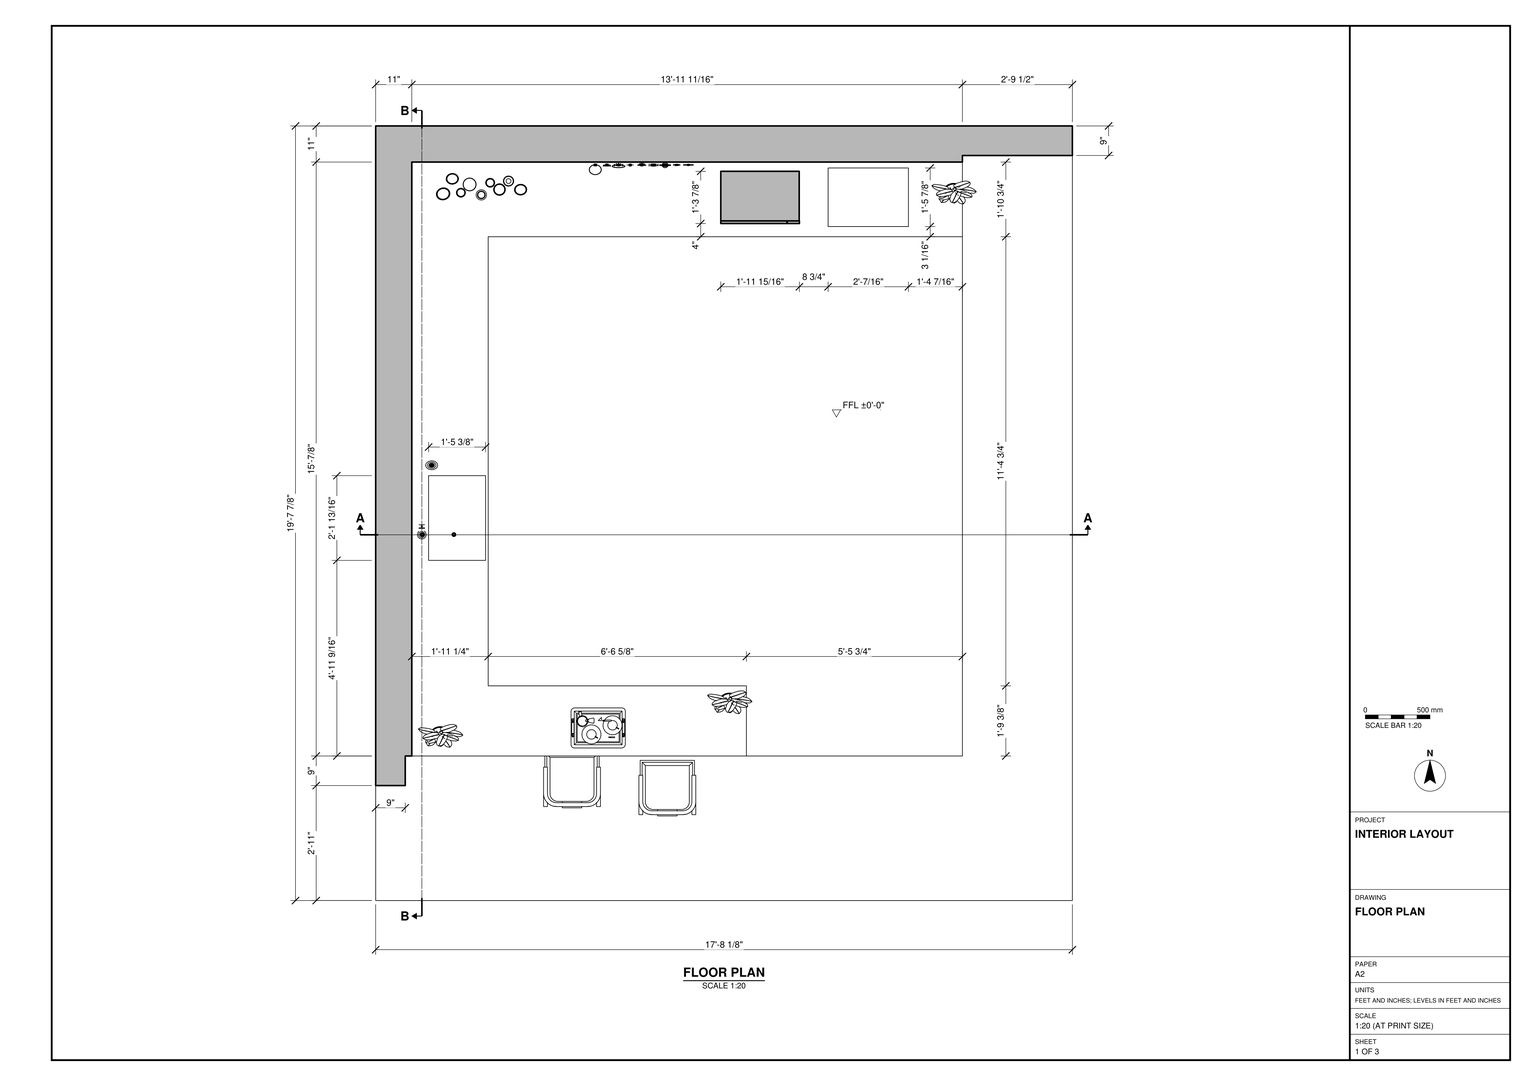
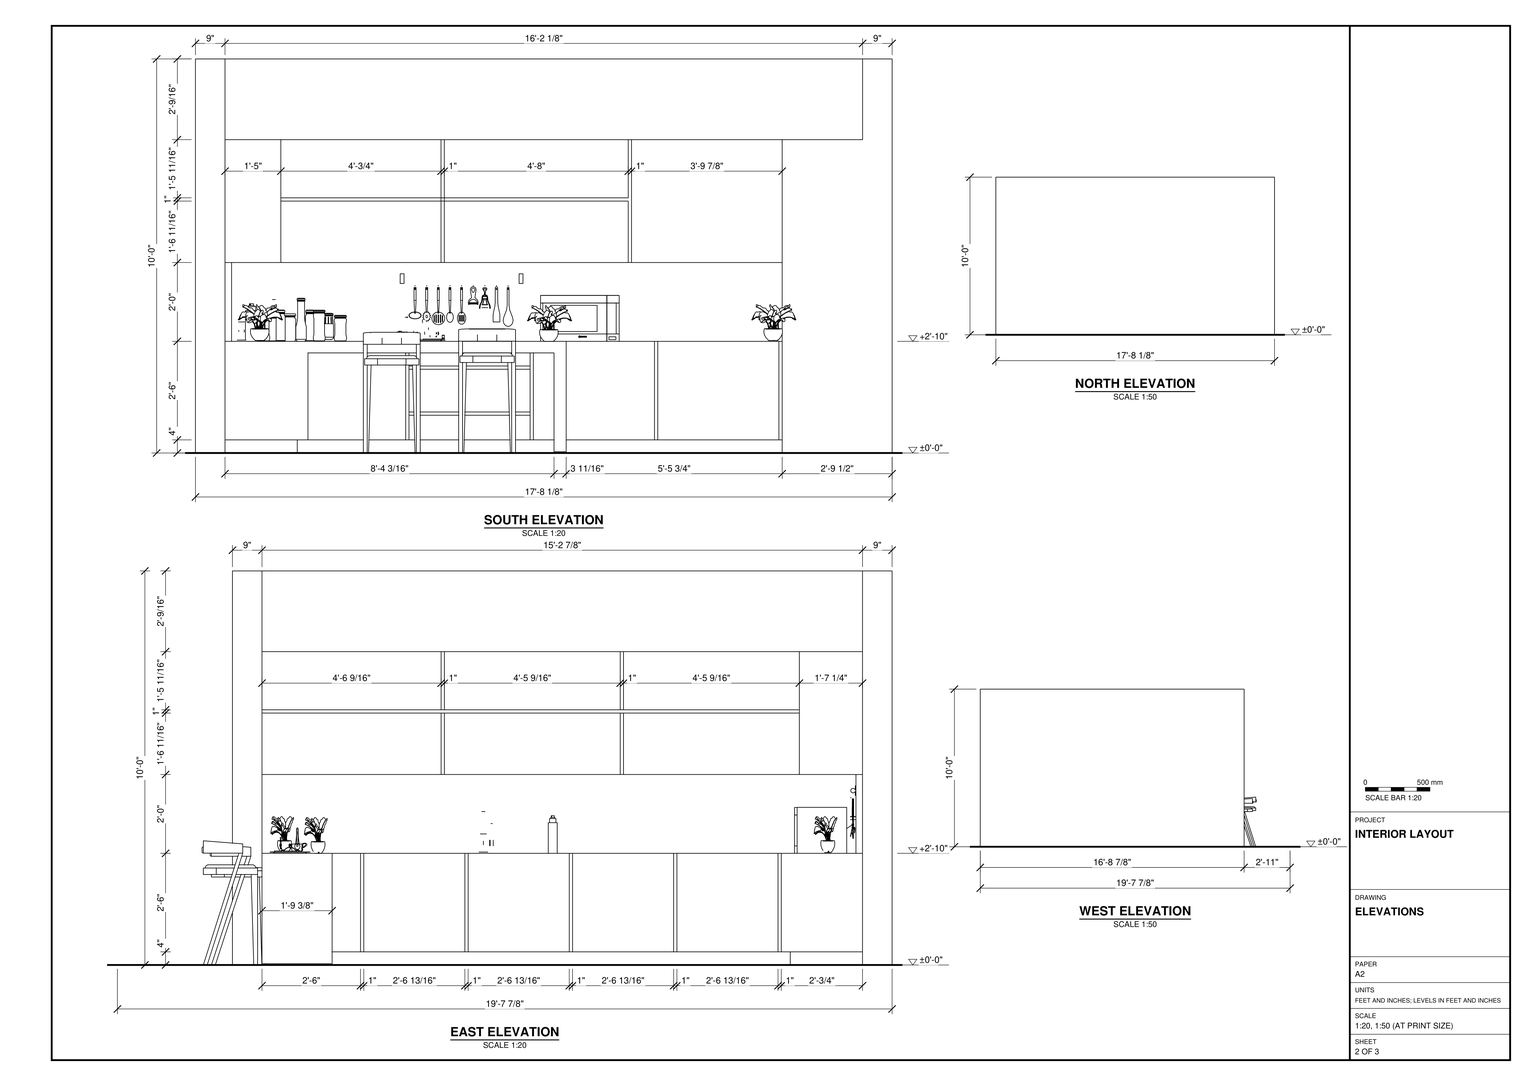
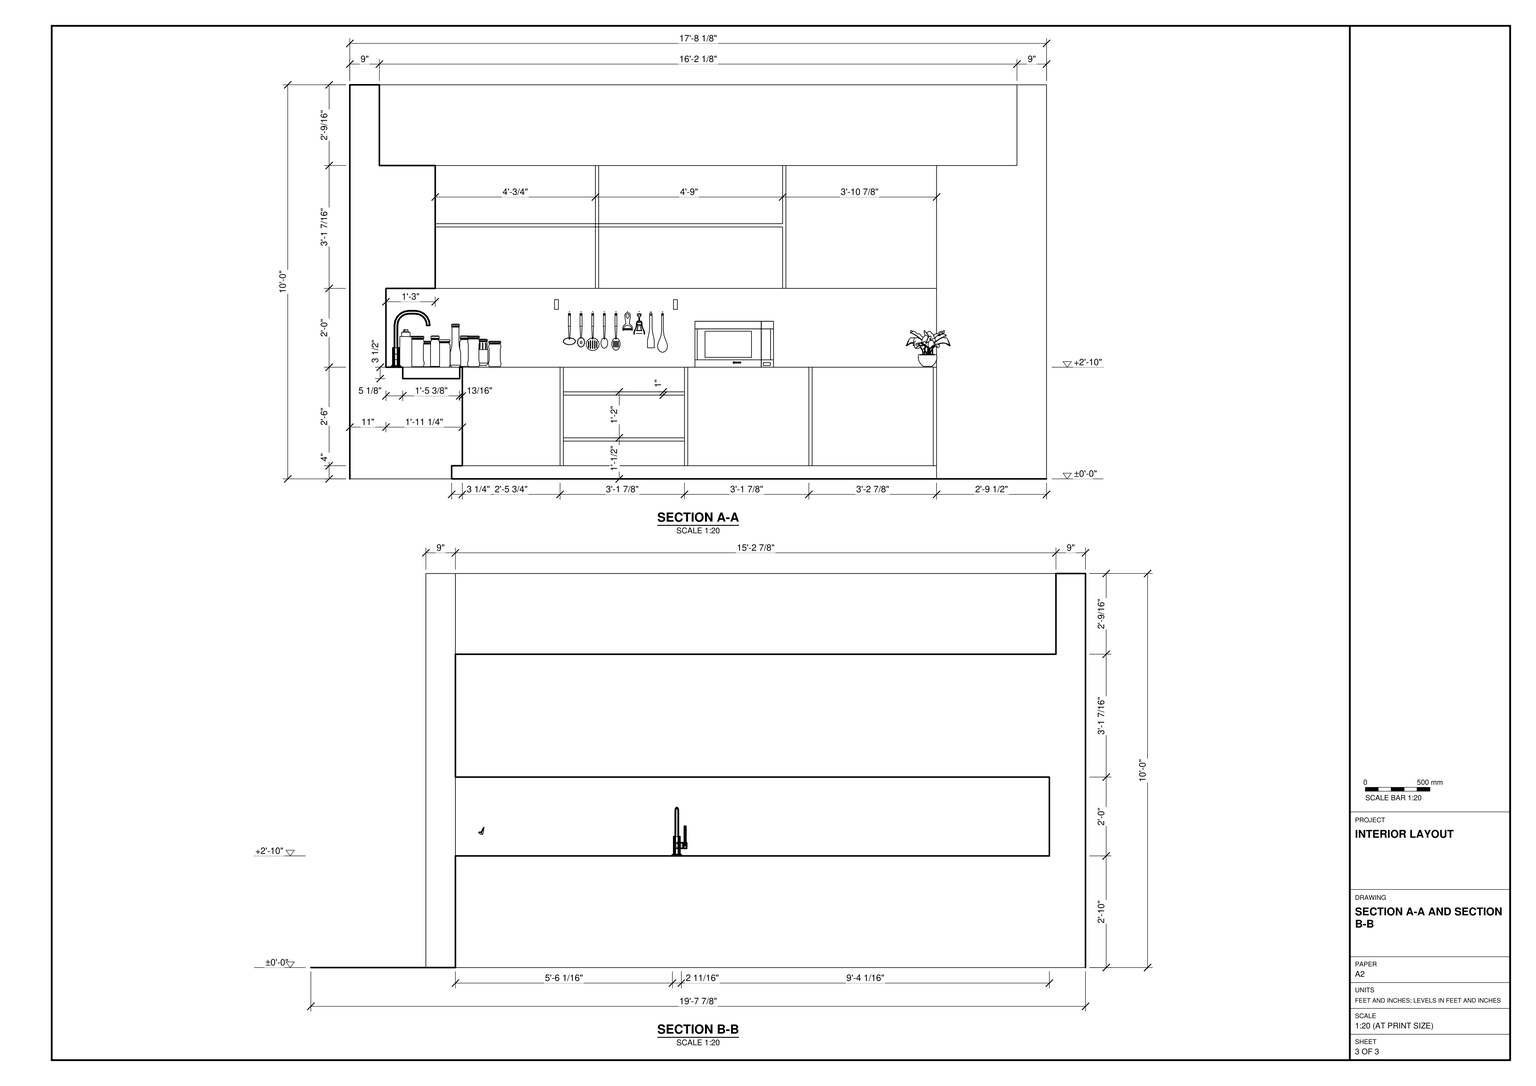
Build the kitchen in SketchUp using task_files/diagram_01.pdf. Work in feet and inches. Set the finished floor at ±0'-0" and make the overall model 17'-8 1/8" east to west, 19'-7 7/8" north to south and 10'-0" high. Model the rectangular floor and the north and west walls. Follow the wall profiles in plan, including the 11" thicknesses beside the counters and the 9" thicknesses at the exposed ends. Leave the south and east sides open as drawn.

Run the base cabinets and worktops along the two walls. Set the worktops at +2'-10" and fit the rectangular sink and tap into the west run. Use the elevations and sections to lay out the recessed plinths, cabinet divisions, shelved bay and shallower upper units. Place the microwave on the north worktop and the hanging utensils in the space below the upper units. Turn the south end of the west worktop into a breakfast peninsula with an end support. Place two stools along its south edge, leaving access to the kitchen around its east end.

Decor and loose items, including plants, tableware, utensils and appliances, may be any suitable library components. Keep the floor, walls and individual furniture and joinery pieces in separate groups or components, and use components for repeated parts. Save one SketchUp model as output_files/corner_kitchen_with_a_breakfast_peninsula.skp.

# SketchUp Ruby script. Lengths in inches.
U = 1.inch
M = Sketchup.active_model
def pt(a) = Geom::Point3d.new(a.map { |v| v * U })
def face(e, loops, mat)
  f = e.add_face(loops[0].map { |a| pt(a) })
  loops[1..].each { |l| e.add_face(l.map { |a| pt(a) }).erase! }
  f.material = f.back_material = mat if mat
  f
end
# faces: each face lists its corners as indices into pts; further lists are holes
def faces(e, pts, list, mat = nil) = list.each { |f| face(e, (f[0].is_a?(Array) ? f : [f]).map { |l| l.map { |i| pts[i] } }, mat) }
# xy, xz, yz: faces in a plane at the given z, y or x. An outline is a flat list of corners, or four numbers for a rectangle; further outlines are holes
def ring(l) = l.size == 4 ? [[l[0], l[1]], [l[2], l[1]], [l[2], l[3]], [l[0], l[3]]] : l.each_slice(2).to_a
def flat(e, list, mat, &to3) = list.each { |f| face(e, (f[0].is_a?(Array) ? f : [f]).map { |l| ring(l).map { |u, v| to3.(u, v) } }, mat) }
def xy(e, z, list, mat = nil) = flat(e, list, mat) { |x, y| [x, y, z] }
def xz(e, y, list, mat = nil) = flat(e, list, mat) { |x, z| [x, y, z] }
def yz(e, x, list, mat = nil) = flat(e, list, mat) { |y, z| [x, y, z] }
def lines(e, pts, list) = list.each { |a, b| e.add_line(pt(pts[a]), pt(pts[b])) }
# prism: a flat outline (further loops are holes) pulled along v
def prism(e, loops, v, mat = nil)
  f = face(e, loops, mat); d = Geom::Vector3d.new(v.map { |x| x * U })
  f.pushpull(f.normal.samedirection?(d) ? d.length : -d.length)
end
def box(e, o, s, mat = nil) = prism(e, [[o, [o[0] + s[0], o[1], o[2]], [o[0] + s[0], o[1] + s[1], o[2]], [o[0], o[1] + s[1], o[2]]]], [0, 0, s[2]], mat)
def at(x, y, z, deg = 0) = Geom::Transformation.translation(pt([x, y, z])) * Geom::Transformation.rotation(ORIGIN, Z_AXIS, deg.degrees)
def axes(o, x, y, z) = Geom::Transformation.new([*x, 0, *y, 0, *z, 0, *pt(o).to_a, 1])
def part(name) = M.definitions.add(name)
# library, detail: a bought-in or finely detailed component or shape, given as its bounding box
def library(name, o, s) = part(name).tap { |d| box(d.entities, o, s) }
def detail(e, o, s) = box(e.add_group.entities, o, s)
def put(e, d, t, mat = nil) = e.add_instance(d, t).tap { |i| i.material = mat if mat }
def group(e, t, mat = nil) = e.add_group.tap { |g| g.transformation = t; g.material = mat if mat }.entities
root = M.entities
M.materials.add("Marble_06_1K").color = [165, 150, 147]
M.materials.add("Marble_07_1K").color = [36, 34, 36]
M.materials.add("Plywood_08_1K").color = [202, 166, 113]
c1 = library("Kitchen Tap",[-1.36,-10.33,0],[4.36,11.69,17.22])
c2 = library("bar stool",[-2.36,0,0],[17.32,16.92,37.82])
c3 = library("flowers vase",[54.24,177.42,-0.18],[13.15,11.36,9.96])
c4 = library("Encurtidos",[-8.17,-2.25,0],[16.27,5.07,6.57])
c5 = part("hand_cream")
prism(c5.entities,[[[-1443.3125,-20.9,1754.4],[-1443.21,-20.95,1753.51],[-1443.3125,-20.9,1752.63],[-1443.61,-20.73,1751.81],[-1444.09,-20.47,1751.1],[-1444.7,-20.13,1750.5625],[-1445.43,-19.74,1750.22],[-1446.2,-19.3125,1750.1],[-1446.97,-18.89,1750.22],[-1447.69,-18.49,1750.5625],[-1448.3125,-18.15,1751.1],[-1448.79,-17.89,1751.81],[-1449.09,-17.73,1752.63],[-1449.1875,-17.67,1753.51],[-1449.09,-17.73,1754.4],[-1448.79,-17.89,1755.22],[-1448.3125,-18.15,1755.92],[-1447.69,-18.49,1756.47],[-1446.97,-18.89,1756.81],[-1446.2,-19.3125,1756.92],[-1445.43,-19.74,1756.81],[-1444.7,-20.13,1756.47],[-1444.09,-20.47,1755.92],[-1443.61,-20.73,1755.22]]],[-4.29,-7.82,0])
xy(c5.entities,0,[[[-1381.3,-265.26,-1467.95,-252.53,-1548.36,-217.8,-1617.03,-163.45,-1669.3,-93.17,-1701.6,-11.76,-1711.73,75.24,-1698.99,161.89,-1664.27,242.29,-1609.91,310.97,-1539.64,363.24,-1458.23,395.54,-1371.23,405.66,-1284.58,392.93,-1204.17,358.2,-1135.5,303.85,-1083.23,233.57,-1050.93,152.16,-1040.8,65.17,-1053.54,-21.49,-1088.26,-101.89,-1142.62,-170.57,-1212.9,-222.84,-1294.31,-255.13],[-1376.27,57.7,-1373.03,58.125,-1370.02,59.375,-1367.43,61.36,-1365.44,63.95,-1364.19,66.97,-1363.77,70.2,-1364.19,73.4375,-1365.44,76.45,-1367.43,79.04,-1370.02,81.03,-1373.03,82.27,-1376.27,82.7,-1379.5,82.27,-1382.52,81.03,-1385.1,79.04,-1387.09,76.45,-1388.34,73.4375,-1388.77,70.2,-1388.34,66.97,-1387.09,63.95,-1385.1,61.36,-1382.52,59.375,-1379.5,58.125]]])
xy(c5.entities,1460,[[[-1381.3,-265.26,-1294.31,-255.13,-1212.9,-222.84,-1142.62,-170.57,-1088.26,-101.89,-1053.54,-21.49,-1040.8,65.17,-1050.93,152.16,-1083.23,233.57,-1135.5,303.85,-1204.17,358.2,-1284.58,392.93,-1371.23,405.66,-1458.23,395.54,-1539.64,363.24,-1609.91,310.97,-1664.27,242.29,-1698.99,161.89,-1711.73,75.24,-1701.6,-11.76,-1669.3,-93.17,-1617.03,-163.45,-1548.36,-217.8,-1467.95,-252.53],[-1389.27,-168.95,-1450.72,-157.43,-1507.1,-130.4,-1554.56,-89.7,-1589.875,-38.11,-1610.63,20.87,-1615.41,83.21,-1603.9,144.66,-1576.87,201.04,-1536.17,248.5,-1484.58,283.8125,-1425.6,304.56,-1363.26,309.35,-1301.81,297.83,-1245.43,270.8,-1197.97,230.11,-1162.66,178.51,-1141.9,119.53,-1137.12,57.19,-1148.63,-4.26,-1175.66,-60.64,-1216.36,-108.1,-1267.96,-143.41,-1326.93,-164.16]]])
xy(c5.entities,1656,[[[-1389.27,-168.95,-1326.93,-164.16,-1267.96,-143.41,-1216.36,-108.1,-1175.66,-60.64,-1148.63,-4.26,-1137.12,57.19,-1141.9,119.53,-1162.66,178.51,-1197.97,230.11,-1245.43,270.8,-1301.81,297.83,-1363.26,309.35,-1425.6,304.56,-1484.58,283.8125,-1536.17,248.5,-1576.87,201.04,-1603.9,144.66,-1615.41,83.21,-1610.63,20.87,-1589.875,-38.11,-1554.56,-89.7,-1507.1,-130.4,-1450.72,-157.43],[-1362.32,-87.43,-1403.59,-85.67,-1443,-73.29,-1477.87,-51.125,-1505.81,-20.7,-1524.92,15.93,-1533.9,56.25,-1532.14,97.53,-1519.76,136.9375,-1497.59,171.8,-1467.16,199.74,-1430.54,218.85,-1390.21,227.83,-1348.94,226.07,-1309.53,213.69,-1274.66,191.53,-1246.72,161.1,-1227.61,124.47,-1218.63,84.15,-1220.39,42.875,-1232.78,3.46,-1254.9375,-31.4,-1285.37,-59.34,-1321.99,-78.45]]])
xy(c5.entities,1706.5,[[[-1362.32,-87.43,-1321.99,-78.45,-1285.37,-59.34,-1254.9375,-31.4,-1232.78,3.46,-1220.39,42.875,-1218.63,84.15,-1227.61,124.47,-1246.72,161.1,-1274.66,191.53,-1309.53,213.69,-1348.94,226.07,-1390.21,227.83,-1430.54,218.85,-1467.16,199.74,-1497.59,171.8,-1519.76,136.9375,-1532.14,97.53,-1533.9,56.25,-1524.92,15.93,-1505.81,-20.7,-1477.87,-51.125,-1443,-73.29,-1403.59,-85.67],[-1388.64,-43.125,-1417.55,-36.06,-1443.65,-21.75,-1465.15,-1.18,-1480.6,24.26,-1488.93,52.83,-1489.59,82.58,-1482.53,111.49,-1468.22,137.58,-1447.65,159.09,-1422.21,174.53,-1393.64,182.87,-1363.89,183.53,-1334.98,176.46,-1308.88,162.15,-1287.38,141.58,-1271.93,116.14,-1263.6,87.57,-1262.94,57.82,-1270.01,28.91,-1284.3125,2.82,-1304.89,-18.6875,-1330.32,-34.13,-1358.89,-42.47]]])
xy(c5.entities,1791,[[-1399.18,45.73,-1328.74,45.73,-1399.18,105.97]])
xy(c5.entities,1791.5,[[[-1388.64,-43.125,-1358.89,-42.47,-1330.32,-34.13,-1304.89,-18.6875,-1284.3125,2.82,-1270.01,28.91,-1262.94,57.82,-1263.6,87.57,-1271.93,116.14,-1287.38,141.58,-1308.88,162.15,-1334.98,176.46,-1363.89,183.53,-1393.64,182.87,-1422.21,174.53,-1447.65,159.09,-1468.22,137.58,-1482.53,111.49,-1489.59,82.58,-1488.93,52.83,-1480.6,24.26,-1465.15,-1.18,-1443.65,-21.75,-1417.55,-36.06],[-1365.03,-21.65,-1398.96,-16.68,-1428.71,0.36,-1450.16,27.11,-1460.32,59.86,-1457.79,94.05,-1442.91,124.95,-1417.75,148.25,-1385.8125,160.72,-1276.95,67.61,-1284.3125,34.12,-1303.43,5.65,-1331.64,-13.84]],[[-1365.03,-21.65,-1331.64,-13.84,-1303.43,5.65,-1284.3125,34.12,-1276.95,67.61,-1385.8125,160.72,-1417.75,148.25,-1442.91,124.95,-1457.79,94.05,-1460.32,59.86,-1450.16,27.11,-1428.71,0.36,-1398.96,-16.68],[-1399.18,45.73,-1399.18,105.97,-1328.74,45.73],[-1376.27,57.7,-1379.5,58.125,-1382.52,59.375,-1385.1,61.36,-1387.09,63.95,-1388.34,66.97,-1388.77,70.2,-1388.34,73.4375,-1387.09,76.45,-1385.1,79.04,-1382.52,81.03,-1379.5,82.27,-1376.27,82.7,-1373.03,82.27,-1370.02,81.03,-1367.43,79.04,-1365.44,76.45,-1364.19,73.4375,-1363.77,70.2,-1364.19,66.97,-1365.44,63.95,-1367.43,61.36,-1370.02,59.375,-1373.03,58.125]]])
xz(c5.entities,45.73,[[-1399.18,1791,-1328.74,1791.5]])
yz(c5.entities,-1399.18,[[45.73,1791,105.97,1791.5]])
p = [[-1467.95,-252.53,0],[-1381.3,-265.26,0],[-1381.3,-265.26,1460],[-1467.95,-252.53,1460],[-1294.31,-255.13,0],[-1294.31,-255.13,1460],
  [-1212.9,-222.84,0],[-1212.9,-222.84,1460],[-1548.36,-217.8,0],[-1548.36,-217.8,1460],[-1142.62,-170.57,0],[-1142.62,-170.57,1460],
  [-1617.03,-163.45,0],[-1617.03,-163.45,1460],[-1088.26,-101.89,0],[-1088.26,-101.89,1460],[-1669.3,-93.17,0],[-1669.3,-93.17,1460],
  [-1053.54,-21.49,0],[-1053.54,-21.49,1460],[-1701.6,-11.76,0],[-1701.6,-11.76,1460],[-1040.8,65.17,0],[-1040.8,65.17,1460],
  [-1711.73,75.24,0],[-1711.73,75.24,1460],[-1379.5,58.125,1791.5],[-1376.27,57.7,1791.5],[-1376.27,57.7,0],[-1379.5,58.125,0],
  [-1373.03,58.125,1791.5],[-1373.03,58.125,0],[-1382.52,59.375,1791.5],[-1382.52,59.375,0],[-1370.02,59.375,1791.5],[-1370.02,59.375,0],
  [-1385.1,61.36,1791.5],[-1385.1,61.36,0],[-1367.43,61.36,1791.5],[-1367.43,61.36,0],[-1387.09,63.95,1791.5],[-1387.09,63.95,0],
  [-1365.44,63.95,1791.5],[-1365.44,63.95,0],[-1388.34,66.97,1791.5],[-1388.34,66.97,0],[-1364.19,66.97,1791.5],[-1364.19,66.97,0],
  [-1050.93,152.16,0],[-1050.93,152.16,1460],[-1388.77,70.2,1791.5],[-1388.77,70.2,0],[-1363.77,70.2,1791.5],[-1363.77,70.2,0],
  [-1388.34,73.4375,1791.5],[-1388.34,73.4375,0],[-1364.19,73.4375,1791.5],[-1364.19,73.4375,0],[-1387.09,76.45,1791.5],[-1387.09,76.45,0],
  [-1365.44,76.45,1791.5],[-1365.44,76.45,0],[-1698.99,161.89,0],[-1698.99,161.89,1460],[-1385.1,79.04,1791.5],[-1385.1,79.04,0],
  [-1367.43,79.04,1791.5],[-1367.43,79.04,0],[-1382.52,81.03,1791.5],[-1382.52,81.03,0],[-1370.02,81.03,1791.5],[-1370.02,81.03,0],
  [-1379.5,82.27,1791.5],[-1379.5,82.27,0],[-1373.03,82.27,1791.5],[-1373.03,82.27,0],[-1376.27,82.7,1791.5],[-1376.27,82.7,0],
  [-1083.23,233.57,0],[-1083.23,233.57,1460],[-1664.27,242.29,0],[-1664.27,242.29,1460],[-1135.5,303.85,0],[-1135.5,303.85,1460],
  [-1609.91,310.97,0],[-1609.91,310.97,1460],[-1204.17,358.2,0],[-1204.17,358.2,1460],[-1539.64,363.24,0],[-1539.64,363.24,1460],
  [-1284.58,392.93,0],[-1284.58,392.93,1460],[-1458.23,395.54,0],[-1458.23,395.54,1460],[-1371.23,405.66,0],[-1371.23,405.66,1460],
  [-1450.72,-157.43,1460],[-1389.27,-168.95,1460],[-1389.27,-168.95,1656],[-1450.72,-157.43,1656],[-1326.93,-164.16,1460],[-1326.93,-164.16,1656],
  [-1267.96,-143.41,1460],[-1267.96,-143.41,1656],[-1507.1,-130.4,1460],[-1507.1,-130.4,1656],[-1216.36,-108.1,1460],[-1216.36,-108.1,1656],
  [-1554.56,-89.7,1460],[-1554.56,-89.7,1656],[-1175.66,-60.64,1460],[-1175.66,-60.64,1656],[-1589.875,-38.11,1460],[-1589.875,-38.11,1656],
  [-1148.63,-4.26,1460],[-1148.63,-4.26,1656],[-1610.63,20.87,1460],[-1610.63,20.87,1656],[-1137.12,57.19,1460],[-1137.12,57.19,1656],
  [-1615.41,83.21,1460],[-1615.41,83.21,1656],[-1141.9,119.53,1460],[-1141.9,119.53,1656],[-1603.9,144.66,1460],[-1603.9,144.66,1656],
  [-1162.66,178.51,1460],[-1162.66,178.51,1656],[-1576.87,201.04,1460],[-1576.87,201.04,1656],[-1197.97,230.11,1460],[-1197.97,230.11,1656],
  [-1536.17,248.5,1460],[-1536.17,248.5,1656],[-1245.43,270.8,1460],[-1245.43,270.8,1656],[-1484.58,283.8125,1460],[-1484.58,283.8125,1656],
  [-1301.81,297.83,1460],[-1301.81,297.83,1656],[-1425.6,304.56,1460],[-1425.6,304.56,1656],[-1363.26,309.35,1460],[-1363.26,309.35,1656],
  [-1403.59,-85.67,1656],[-1362.32,-87.43,1656],[-1362.32,-87.43,1706.5],[-1403.59,-85.67,1706.5],[-1321.99,-78.45,1656],[-1321.99,-78.45,1706.5],
  [-1443,-73.29,1656],[-1443,-73.29,1706.5],[-1285.37,-59.34,1656],[-1285.37,-59.34,1706.5],[-1477.87,-51.125,1656],[-1477.87,-51.125,1706.5],
  [-1254.9375,-31.4,1656],[-1254.9375,-31.4,1706.5],[-1505.81,-20.7,1656],[-1505.81,-20.7,1706.5],[-1232.78,3.46,1656],[-1232.78,3.46,1706.5],
  [-1524.92,15.93,1656],[-1524.92,15.93,1706.5],[-1220.39,42.875,1656],[-1220.39,42.875,1706.5],[-1533.9,56.25,1656],[-1533.9,56.25,1706.5],
  [-1218.63,84.15,1656],[-1218.63,84.15,1706.5],[-1532.14,97.53,1656],[-1532.14,97.53,1706.5],[-1227.61,124.47,1656],[-1227.61,124.47,1706.5],
  [-1519.76,136.9375,1656],[-1519.76,136.9375,1706.5],[-1246.72,161.1,1656],[-1246.72,161.1,1706.5],[-1497.59,171.8,1656],[-1497.59,171.8,1706.5],
  [-1274.66,191.53,1656],[-1274.66,191.53,1706.5],[-1467.16,199.74,1656],[-1467.16,199.74,1706.5],[-1309.53,213.69,1656],[-1309.53,213.69,1706.5],
  [-1430.54,218.85,1656],[-1430.54,218.85,1706.5],[-1348.94,226.07,1656],[-1348.94,226.07,1706.5],[-1390.21,227.83,1656],[-1390.21,227.83,1706.5],
  [-1417.55,-36.06,1706.5],[-1388.64,-43.125,1706.5],[-1388.64,-43.125,1791.5],[-1417.55,-36.06,1791.5],[-1358.89,-42.47,1706.5],[-1358.89,-42.47,1791.5],
  [-1330.32,-34.13,1706.5],[-1330.32,-34.13,1791.5],[-1443.65,-21.75,1706.5],[-1443.65,-21.75,1791.5],[-1304.89,-18.6875,1706.5],[-1304.89,-18.6875,1791.5],
  [-1465.15,-1.18,1706.5],[-1465.15,-1.18,1791.5],[-1284.3125,2.82,1706.5],[-1284.3125,2.82,1791.5],[-1480.6,24.26,1706.5],[-1480.6,24.26,1791.5],
  [-1270.01,28.91,1706.5],[-1270.01,28.91,1791.5],[-1488.93,52.83,1706.5],[-1488.93,52.83,1791.5],[-1262.94,57.82,1706.5],[-1262.94,57.82,1791.5],
  [-1489.59,82.58,1706.5],[-1489.59,82.58,1791.5],[-1263.6,87.57,1706.5],[-1263.6,87.57,1791.5],[-1482.53,111.49,1706.5],[-1482.53,111.49,1791.5],
  [-1271.93,116.14,1706.5],[-1271.93,116.14,1791.5],[-1468.22,137.58,1706.5],[-1468.22,137.58,1791.5],[-1287.38,141.58,1706.5],[-1287.38,141.58,1791.5],
  [-1447.65,159.09,1706.5],[-1447.65,159.09,1791.5],[-1308.88,162.15,1706.5],[-1308.88,162.15,1791.5],[-1422.21,174.53,1706.5],[-1422.21,174.53,1791.5],
  [-1334.98,176.46,1706.5],[-1334.98,176.46,1791.5],[-1393.64,182.87,1706.5],[-1393.64,182.87,1791.5],[-1363.89,183.53,1706.5],[-1363.89,183.53,1791.5],
  [-1425.87,-47.07,1753.51],[-1426.7,-46.27,1762.28],[-1429.15,-43.93,1770.45],[-1433.04,-40.21,1777.47],[-1438.11,-35.36,1782.85],[-1444.01,-29.71,1786.23],
  [-1450.35,-23.65,1787.39],[-1456.68,-17.59,1786.23],[-1462.59,-11.94,1782.85],[-1467.65,-7.09,1777.47],[-1471.54,-3.37,1770.45],[-1473.99,-1.03,1762.28],
  [-1474.82,-0.23,1753.51],[-1473.99,-1.03,1744.75],[-1471.54,-3.37,1736.58],[-1467.65,-7.09,1729.5625],[-1462.59,-11.94,1724.18],[-1456.68,-17.59,1720.79],
  [-1450.35,-23.65,1719.64],[-1444.01,-29.71,1720.79],[-1438.11,-35.36,1724.18],[-1433.04,-40.21,1729.5625],[-1429.15,-43.93,1736.58],[-1426.7,-46.27,1744.75],
  [-1440.21,-33.34,1764.8],[-1438.45,-35.03,1760.78],[-1437.49,-35.95,1756.27],[-1437.42,-36.02,1751.57],[-1438.22,-35.25,1747.01],[-1439.85,-33.69,1742.89],
  [-1442.2,-31.45,1739.49],[-1445.1,-28.67,1737.05],[-1448.35,-25.56,1735.73],[-1451.75,-22.31,1735.62],[-1455.05,-19.15,1736.73],[-1458.03,-16.3,1738.99],
  [-1460.48,-13.95,1742.23],[-1462.25,-12.26,1746.25],[-1463.2,-11.35,1750.76],[-1463.28,-11.28,1755.45],[-1462.47,-12.05,1760.02],[-1460.84,-13.61,1764.14],
  [-1458.5,-15.85,1767.54],[-1455.6,-18.625,1769.98],[-1452.34,-21.74,1771.3],[-1448.95,-24.99,1771.41],[-1445.65,-28.15,1770.3],[-1442.67,-31,1768.04],
  [-1422.56,-41.93,1762.28],[-1421.72,-42.73,1753.51],[-1422.56,-41.93,1744.75],[-1425,-39.59,1736.58],[-1428.89,-35.87,1729.5625],[-1433.96,-31.02,1724.18],
  [-1439.86,-25.375,1720.79],[-1446.2,-19.3125,1719.64],[-1452.53,-13.25,1720.79],[-1458.4375,-7.6,1724.18],[-1463.51,-2.75,1729.5625],[-1467.4,0.97,1736.58],
  [-1469.84,3.31,1744.75],[-1470.68,4.1,1753.51],[-1469.84,3.31,1762.28],[-1467.4,0.97,1770.45],[-1463.51,-2.75,1777.47],[-1458.4375,-7.6,1782.85],
  [-1452.53,-13.25,1786.23],[-1446.2,-19.3125,1787.39],[-1439.86,-25.375,1786.23],[-1433.96,-31.02,1782.85],[-1428.89,-35.87,1777.47],[-1425,-39.59,1770.45],
  [-1434.3,-30.7,1760.78],[-1436.06,-29.01,1764.8],[-1438.52,-26.66,1768.04],[-1441.5,-23.8125,1770.3],[-1444.8,-20.65,1771.41],[-1448.19,-17.41,1771.3],
  [-1451.45,-14.29,1769.98],[-1454.35,-11.51,1767.54],[-1456.7,-9.27,1764.14],[-1458.33,-7.71,1760.02],[-1459.13,-6.94,1755.45],[-1459.05,-7.02,1750.76],
  [-1458.1,-7.93,1746.25],[-1456.33,-9.62,1742.23],[-1453.88,-11.97,1738.99],[-1450.9,-14.82,1736.73],[-1447.6,-17.97,1735.62],[-1444.21,-21.22,1735.73],
  [-1440.95,-24.34,1737.05],[-1438.05,-27.11,1739.49],[-1435.7,-29.36,1742.89],[-1434.07,-30.92,1747.01],[-1433.27,-31.68,1751.57],[-1433.35,-31.61,1756.27],
  [-1328.74,45.73,1791.5],[-1399.18,105.97,1791.5],[-1399.18,105.97,1791],[-1328.74,45.73,1791],[-1391.1,151.05,1791.5],[-1293.54,67.61,1791.5],
  [-1405.55,141.52,1791.5],[-1293.54,45.73,1791.5],[-1415.9,133.2,1791.5],[-1300.19,34.25,1791.5],[-1428.65,118.89,1791.5],[-1409.14,95.77,1791.5],
  [-1344.88,33.9375,1791.5],[-1311.85,14.66,1791.5],[-1437.11,102.52,1791.5],[-1407.04,67.37,1791.5],[-1372.23,38.25,1791.5],[-1329.53,6.85,1791.5],
  [-1445.99,88.67,1791.5],[-1344.39,-2.86,1791.5],[-1447.2,74.64,1791.5],[-1361.18,-2.86,1791.5],[-1449.95,61.33,1791.5],[-1372.23,-8.68,1791.5],
  [-1439.43,35.99,1791.5],[-1389.84,-8.68,1791.5]]
faces(c5.entities,p,[[0,1,2,3],[1,4,5,2],[4,6,7,5],[8,0,3,9],[6,10,11,7],[12,8,9,13],[10,14,15,11],[16,12,13,17],
  [14,18,19,15],[20,16,17,21],[18,22,23,19],[24,20,21,25],[26,27,28,29],[27,30,31,28],[32,26,29,33],[30,34,35,31],
  [36,32,33,37],[34,38,39,35],[40,36,37,41],[38,42,43,39],[44,40,41,45],[42,46,47,43],[22,48,49,23],[50,44,45,51],
  [46,52,53,47],[54,50,51,55],[52,56,57,53],[58,54,55,59],[56,60,61,57],[62,24,25,63],[64,58,59,65],[60,66,67,61],
  [68,64,65,69],[66,70,71,67],[72,68,69,73],[70,74,75,71],[76,72,73,77],[74,76,77,75],[48,78,79,49],[80,62,63,81],
  [78,82,83,79],[84,80,81,85],[82,86,87,83],[88,84,85,89],[86,90,91,87],[92,88,89,93],[90,94,95,91],[94,92,93,95],
  [96,97,98,99],[97,100,101,98],[100,102,103,101],[104,96,99,105],[102,106,107,103],[108,104,105,109],[106,110,111,107],[112,108,109,113],
  [110,114,115,111],[116,112,113,117],[114,118,119,115],[120,116,117,121],[118,122,123,119],[124,120,121,125],[122,126,127,123],[128,124,125,129],
  [126,130,131,127],[132,128,129,133],[130,134,135,131],[136,132,133,137],[134,138,139,135],[140,136,137,141],[138,142,143,139],[142,140,141,143],
  [144,145,146,147],[145,148,149,146],[150,144,147,151],[148,152,153,149],[154,150,151,155],[152,156,157,153],[158,154,155,159],[156,160,161,157],
  [162,158,159,163],[160,164,165,161],[166,162,163,167],[164,168,169,165],[170,166,167,171],[168,172,173,169],[174,170,171,175],[172,176,177,173],
  [178,174,175,179],[176,180,181,177],[182,178,179,183],[180,184,185,181],[186,182,183,187],[184,188,189,185],[190,186,187,191],[188,190,191,189],
  [192,193,194,195],[193,196,197,194],[196,198,199,197],[200,192,195,201],[198,202,203,199],[204,200,201,205],[202,206,207,203],[208,204,205,209],
  [206,210,211,207],[212,208,209,213],[210,214,215,211],[216,212,213,217],[214,218,219,215],[220,216,217,221],[218,222,223,219],[224,220,221,225],
  [222,226,227,223],[228,224,225,229],[226,230,231,227],[232,228,229,233],[230,234,235,231],[236,232,233,237],[234,238,239,235],[238,236,237,239],
  [[240,241,242,243,244,245,246,247,248,249,250,251,252,253,254,255,256,257,258,259,260,261,262,263],[264,265,266,267,268,269,270,271,272,273,274,275,276,277,278,279,280,281,282,283,284,285,286,287]],[[288,289,290,291,292,293,294,295,296,297,298,299,300,301,302,303,304,305,306,307,308,309,310,311],[312,313,314,315,316,317,318,319,320,321,322,323,324,325,326,327,328,329,330,331,332,333,334,335]],[295,294,259,258],[296,295,258,257],[294,293,260,259],[297,296,257,256],[293,292,261,260],[298,297,256,255],
  [292,291,262,261],[299,298,255,254],[264,265,266,267,268,269,270,271,272,273,274,275,276,277,278,279,280,281,282,283,284,285,286,287],[272,329,328,273],[273,328,327,274],[271,330,329,272],[291,290,263,262],[300,299,254,253],
  [274,327,326,275],[270,331,330,271],[275,326,325,276],[269,332,331,270],[276,325,324,277],[268,333,332,269],[290,289,240,263],[301,300,253,252],
  [277,324,323,278],[267,334,333,268],[278,323,322,279],[266,335,334,267],[289,288,241,240],[302,301,252,251],[279,322,321,280],[335,312,265,266],
  [280,321,320,281],[264,313,312,265],[288,311,242,241],[303,302,251,250],[281,320,319,282],[313,314,287,264],[282,319,318,283],[286,315,314,287],
  [283,318,317,284],[285,316,315,286],[311,310,243,242],[304,303,250,249],[284,317,316,285],[310,309,244,243],[305,304,249,248],[309,308,245,244],
  [306,305,248,247],[308,307,246,245],[307,306,247,246],[336,337,338,339]])
lines(c5.entities,p,[[340,341],[342,343],[344,345],[346,347],[348,349],[350,351],[352,353],[354,355],[356,357],[358,359],[360,361]])
c6 = library("Kitchen Utensils",[-18.7,-3.84,-14.5625],[37.4,3.84,16.04])
c7 = library("Bosch-Microwave-Oven-HMB5061",[0,0,0],[23.9375,19.875,14])
c8 = library("Tea service tray",[-6.99,-6.32,0],[16.65,12.2,7.74])
xy(root,0,[[31,44.02,178.66,204.89]])
xy(root,0,[[0,0,212.14,0,212.14,226.89,178.66,226.89,178.66,44.02,9,44.02,9,35.02,0,35.02]],"Plywood_08_1K")
xy(root,0.375,[[109.1875,44.02,112.88,65.38]])
xy(root,4,[[31,44.02,34.26,204.89],[34.26,202.15,178.66,204.89]])
xy(root,30.48,[[34.26,44.02,109.1875,65.38]])
xy(root,30.53,[[16.11,103.6,33.47,129.4]],"Marble_07_1K")
xy(root,34,[[137.77,205.25,162.22,223.09]],"Marble_07_1K")
xy(root,34,[[[11,44.02,112.88,44.02,112.88,65.38,34.26,65.38,34.26,202.15,178.66,202.15,178.66,224.89,11,224.89],[16.11,103.6,33.47,129.4],[137.77,205.25,162.22,223.09]]],"Plywood_08_1K")
xy(root,58,[[11,44.02,26,224.89],[26,207.65,178.66,224.89]],"Plywood_08_1K")
xy(root,95.42,[[9,44.02,26,44.02,26,207.65,178.66,207.65,178.66,226.89,9,226.89]],"Plywood_08_1K")
xy(root,120,[[0,35.02,9,35.02,9,226.89,212.14,226.89,212.14,235.89,0,235.89]])
xz(root,35.02,[[0,0,9,120]])
xz(root,44.02,[[109.1875,0.375,112.88,0.375,112.88,34,9,34,9,4,34.26,4,34.26,30.48,109.1875,30.48],[9,34,11,58]])
xz(root,44.02,[[9,0,31,4],[9,58,26,95.42]],"Plywood_08_1K")
xz(root,65.38,[[109.1875,0.375,109.1875,30.48,34.26,30.48,34.26,34,112.88,34,112.88,0.375]])
xz(root,103.6,[[16.11,30.53,33.47,34]],"Marble_07_1K")
xz(root,129.4,[[16.11,30.53,33.47,34]],"Marble_07_1K")
xz(root,202.15,[[34.26,4,64.02,34],[65.02,4,101.9,11.5],[102.9,4,139.78,34],[140.78,4,177.66,34],[65.02,12.5,101.9,25.5],
  [65.02,26.5,101.9,34]])
xz(root,202.15,[[64.02,4,65.02,34],[101.9,4,102.9,34],[139.78,4,140.78,34],[177.66,4,178.66,34],[65.02,11.5,101.9,12.5],
  [65.02,25.5,101.9,26.5]],"Marble_07_1K")
xz(root,204.89,[[31,0,178.66,4]],"Plywood_08_1K")
xz(root,207.65,[[26,58,74.78,76.71],[75.78,58,131.78,76.71],[132.78,58,178.66,95.42],[26,77.71,74.78,95.42],[75.78,77.71,131.78,95.42]])
xz(root,207.65,[[74.78,58,75.78,76.71],[131.78,58,132.78,58,132.78,95.42,131.78,95.42,131.78,77.71,75.78,77.71,75.78,76.71,131.78,76.71],[26,76.71,74.78,77.71],[74.78,76.71,75.78,77.71],[74.78,77.71,75.78,95.42]],"Marble_07_1K")
xz(root,224.89,[[11,34,178.66,58]],"Marble_06_1K")
xz(root,226.89,[[178.66,0,212.14,0,212.14,120,203.14,120,203.14,95.42,178.66,95.42],[9,95.42,203.14,120]])
xz(root,235.89,[[0,0,212.14,120]])
yz(root,0,[[35.02,0,235.89,120]])
yz(root,9,[[35.02,0,44.02,120],[44.02,95.42,226.89,120]])
yz(root,11,[[44.02,34,224.89,58]],"Marble_06_1K")
yz(root,16.11,[[103.6,30.53,129.4,34]],"Marble_07_1K")
yz(root,26,[[44.02,58,98.5625,76.71],[99.5625,58,153.11,76.71],[154.11,58,207.65,76.71],[44.02,77.71,98.5625,95.42],[99.5625,77.71,153.11,95.42],
  [154.11,77.71,207.65,95.42]])
yz(root,26,[[98.5625,58,99.5625,76.71],[153.11,58,154.11,76.71],[44.02,76.71,207.65,77.71],[98.5625,77.71,99.5625,95.42],[153.11,77.71,154.11,95.42]],"Marble_07_1K")
yz(root,31,[[44.02,0,204.89,4]],"Plywood_08_1K")
yz(root,33.47,[[103.6,30.53,129.4,34]],"Marble_07_1K")
yz(root,34.26,[[44.02,4,74.02,4,74.02,34,65.38,34,65.38,30.48,44.02,30.48],[75.02,4,105.8,34],[106.8,4,137.59,34],[138.59,4,169.37,34],[170.37,4,201.15,34]])
yz(root,34.26,[[74.02,4,75.02,34],[105.8,4,106.8,34],[137.59,4,138.59,34],[169.37,4,170.37,34],[201.15,4,202.15,34]],"Marble_07_1K")
yz(root,109.1875,[[44.02,0.375,65.38,30.48]])
yz(root,112.88,[[44.02,0.375,65.38,34]])
yz(root,178.66,[[202.15,4,226.89,34],[224.89,34,226.89,58]])
yz(root,178.66,[[204.89,0,226.89,4],[207.65,58,226.89,95.42]],"Plywood_08_1K")
yz(root,212.14,[[226.89,0,235.89,120]])
put(root,c1,at(14.04,111.44,34,90))
put(root,c2,at(95.11,42.69,0,180))
put(root,c2,axes([66.08,45.16,0],[-1,0,0],[0,-1,0],[0,0,0.972]))
put(root,c3,axes([97.125,32.74,34.24],[1.2947,0,0],[0,1,0],[0,0,1.31]))
put(root,c3,axes([-59.22,-132.71,34.24],[1.2947,0,0],[0,1,0],[0,0,1.31]))
put(root,c3,axes([28.83,-122.49,33.96],[1.2947,0,0],[0,1,0],[0,0,1.31]))
put(root,c4,axes([32.03,217.14,34],[1.71748,0.09302,0],[-0.09161,1.69152,0],[0,0,2]))
put(root,c5,axes([24.56,132.27,34],[0.00545,0,0],[0,0.00405,0],[0,0,0.0064]))
put(root,c6,at(81.04,224.89,53.09))
put(root,c7,axes([105.09,206.17,34],[1,0,0],[0,0.8,0],[0,0,1]))
put(root,c8,at(66.47,52.78,34))
